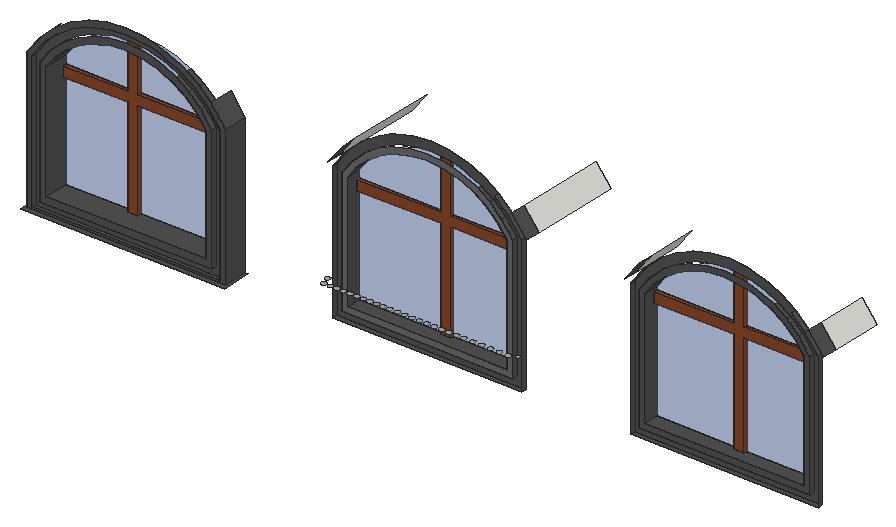
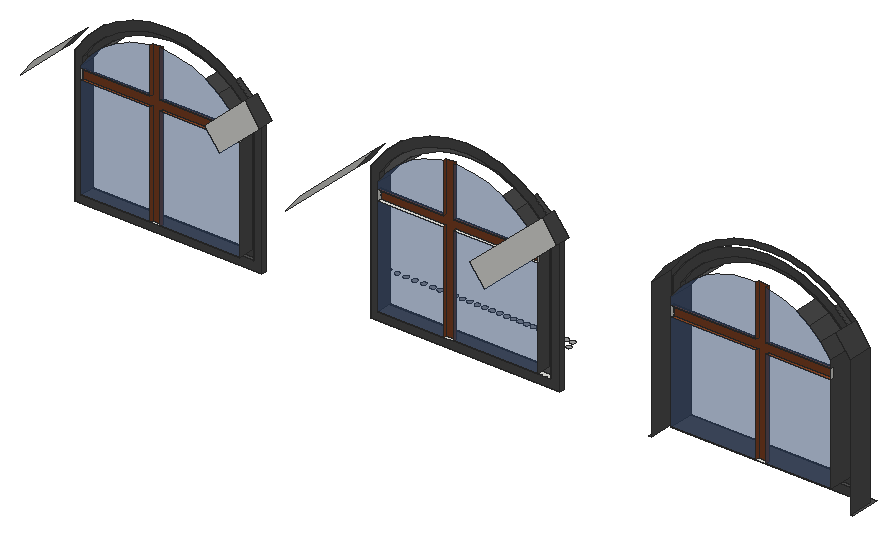
# SketchUp Ruby script. Lengths in inches.
U = 1.inch
M = Sketchup.active_model
def pt(a) = Geom::Point3d.new(a.map { |v| v * U })
def face(e, loops, mat)
  f = e.add_face(loops[0].map { |a| pt(a) })
  loops[1..].each { |l| e.add_face(l.map { |a| pt(a) }).erase! }
  f.material = f.back_material = mat if mat
  f
end
# faces: each face lists its corners as indices into pts; further lists are holes
def faces(e, pts, list, mat = nil) = list.each { |f| face(e, (f[0].is_a?(Array) ? f : [f]).map { |l| l.map { |i| pts[i] } }, mat) }
# xy, xz, yz: faces in a plane at the given z, y or x. An outline is a flat list of corners, or four numbers for a rectangle; further outlines are holes
def ring(l) = l.size == 4 ? [[l[0], l[1]], [l[2], l[1]], [l[2], l[3]], [l[0], l[3]]] : l.each_slice(2).to_a
def flat(e, list, mat, &to3) = list.each { |f| face(e, (f[0].is_a?(Array) ? f : [f]).map { |l| ring(l).map { |u, v| to3.(u, v) } }, mat) }
def xy(e, z, list, mat = nil) = flat(e, list, mat) { |x, y| [x, y, z] }
def xz(e, y, list, mat = nil) = flat(e, list, mat) { |x, z| [x, y, z] }
def yz(e, x, list, mat = nil) = flat(e, list, mat) { |y, z| [x, y, z] }
def lines(e, pts, list) = list.each { |a, b| e.add_line(pt(pts[a]), pt(pts[b])) }
# prism: a flat outline (further loops are holes) pulled along v
def prism(e, loops, v, mat = nil)
  f = face(e, loops, mat); d = Geom::Vector3d.new(v.map { |x| x * U })
  f.pushpull(f.normal.samedirection?(d) ? d.length : -d.length)
end
def box(e, o, s, mat = nil) = prism(e, [[o, [o[0] + s[0], o[1], o[2]], [o[0] + s[0], o[1] + s[1], o[2]], [o[0], o[1] + s[1], o[2]]]], [0, 0, s[2]], mat)
def at(x, y, z, deg = 0) = Geom::Transformation.translation(pt([x, y, z])) * Geom::Transformation.rotation(ORIGIN, Z_AXIS, deg.degrees)
def axes(o, x, y, z) = Geom::Transformation.new([*x, 0, *y, 0, *z, 0, *pt(o).to_a, 1])
def part(name) = M.definitions.add(name)
# library, detail: a bought-in or finely detailed component or shape, given as its bounding box
def library(name, o, s) = part(name).tap { |d| box(d.entities, o, s) }
def detail(e, o, s) = box(e.add_group.entities, o, s)
def put(e, d, t, mat = nil) = e.add_instance(d, t).tap { |i| i.material = mat if mat }
def group(e, t, mat = nil) = e.add_group.tap { |g| g.transformation = t; g.material = mat if mat }.entities
root = M.entities
M.materials.add("[0042_Sienna]").color = [137, 70, 38]
M.materials.add("[0132_LightGray]").color = [169, 169, 169]
M.materials.add("[0134_DimGray]").color = [105, 105, 105]
M.materials.add("[0135_DarkGray]").color = [81, 81, 81]
M.materials.add("[Translucent Glass Blue]").color = [66, 99, 158]
M.materials["[Translucent Glass Blue]"].alpha = 0.5
xy(root,641.05,[[63.64,31.6875,187.39,31.6875,187.39,49.6875,185.57,49.6875,185.57,34.6875,64.89,34.6875,64.89,49.6875,63.64,49.6875]],"[0135_DarkGray]")
xy(root,641.66,[[245.76,40.6875,360.57,43.6875]],"[0135_DarkGray]")
xy(root,641.92,[[68.09,34.6875,182.37,37.6875]],"[0135_DarkGray]")
xy(root,642.07,[[426.42,40.6875,540.41,43.6875]],"[0135_DarkGray]")
xy(root,646.79,[[72.95,34.6875,177.5,37.6875]],"[0135_DarkGray]")
xy(root,647.04,[[251.14,40.6875,355.19,43.6875]])
xy(root,647.27,[[431.625,40.6875,535.21,43.6875]],"[0135_DarkGray]")
xy(root,650.72,[[116.29,47.6875,122.29,49.6875],[305.64,47.6875,311.64,49.6875],[483.7,47.6875,489.7,49.6875]])
xy(root,650.72,[[76.89,34.6875,173.57,34.6875,173.57,49.6875,122.29,49.6875,122.29,47.6875,116.29,47.6875,116.29,49.6875,76.89,49.6875],[254.82,40.6875,351.51,40.6875,351.51,49.6875,311.64,49.6875,311.64,47.6875,305.64,47.6875,305.64,49.6875,254.82,49.6875],[435.07,40.6875,531.76,40.6875,531.76,49.6875,489.7,49.6875,489.7,47.6875,483.7,47.6875,483.7,49.6875,435.07,49.6875]],"[0135_DarkGray]")
xy(root,662.87,[[361.31,35.875,361.57,35.89,361.8125,35.97,362.03,36.11,362.21,36.31,362.32,36.54,362.38,36.8,362.36,37.06,362.28,37.31,362.14,37.52,361.94,37.7,361.71,37.82,361.46,37.87,361.19,37.85,360.95,37.77,360.73,37.63,360.55,37.4375,360.4375,37.2,360.38,36.95,360.4,36.6875,360.48,36.4375,360.62,36.22,360.82,36.05,361.05,35.93]],"[0132_LightGray]")
xy(root,663.85,[[246.33,31.93,246.68,31.97,247.02,32.11,247.3,32.33,247.52,32.62,247.66,32.95,247.7,33.3,247.66,33.66,247.52,33.99,247.3,34.28,247.02,34.49,246.68,34.63,246.33,34.68,245.97,34.63,245.64,34.49,245.36,34.28,245.14,33.99,245,33.66,244.95,33.3,245,32.95,245.14,32.62,245.36,32.33,245.64,32.11,245.97,31.97],[250.33,31.93,250.68,31.97,251.02,32.11,251.3,32.33,251.52,32.62,251.66,32.95,251.7,33.3,251.66,33.66,251.52,33.99,251.3,34.28,251.02,34.49,250.68,34.63,250.33,34.68,249.97,34.63,249.64,34.49,249.36,34.28,249.14,33.99,249,33.66,248.95,33.3,249,32.95,249.14,32.62,249.36,32.33,249.64,32.11,249.97,31.97],[254.33,31.93,254.68,31.97,255.02,32.11,255.3,32.33,255.52,32.62,255.66,32.95,255.7,33.3,255.66,33.66,255.52,33.99,255.3,34.28,255.02,34.49,254.68,34.63,254.33,34.68,253.97,34.63,253.64,34.49,253.36,34.28,253.14,33.99,253,33.66,252.95,33.3,253,32.95,253.14,32.62,253.36,32.33,253.64,32.11,253.97,31.97],[258.33,31.93,258.68,31.97,259.02,32.11,259.3,32.33,259.52,32.62,259.66,32.95,259.7,33.3,259.66,33.66,259.52,33.99,259.3,34.28,259.02,34.49,258.68,34.63,258.33,34.68,257.97,34.63,257.64,34.49,257.36,34.28,257.14,33.99,257,33.66,256.95,33.3,257,32.95,257.14,32.62,257.36,32.33,257.64,32.11,257.97,31.97],[262.33,31.93,262.68,31.97,263.02,32.11,263.3,32.33,263.52,32.62,263.66,32.95,263.7,33.3,263.66,33.66,263.52,33.99,263.3,34.28,263.02,34.49,262.68,34.63,262.33,34.68,261.97,34.63,261.64,34.49,261.36,34.28,261.14,33.99,261,33.66,260.95,33.3,261,32.95,261.14,32.62,261.36,32.33,261.64,32.11,261.97,31.97],
  [266.33,31.93,266.68,31.97,267.02,32.11,267.3,32.33,267.52,32.62,267.66,32.95,267.7,33.3,267.66,33.66,267.52,33.99,267.3,34.28,267.02,34.49,266.68,34.63,266.33,34.68,265.97,34.63,265.64,34.49,265.36,34.28,265.14,33.99,265,33.66,264.95,33.3,265,32.95,265.14,32.62,265.36,32.33,265.64,32.11,265.97,31.97],[270.33,31.93,270.68,31.97,271.02,32.11,271.3,32.33,271.52,32.62,271.66,32.95,271.7,33.3,271.66,33.66,271.52,33.99,271.3,34.28,271.02,34.49,270.68,34.63,270.33,34.68,269.97,34.63,269.64,34.49,269.36,34.28,269.14,33.99,269,33.66,268.95,33.3,269,32.95,269.14,32.62,269.36,32.33,269.64,32.11,269.97,31.97],[274.33,31.93,274.68,31.97,275.02,32.11,275.3,32.33,275.52,32.62,275.66,32.95,275.7,33.3,275.66,33.66,275.52,33.99,275.3,34.28,275.02,34.49,274.68,34.63,274.33,34.68,273.97,34.63,273.64,34.49,273.36,34.28,273.14,33.99,273,33.66,272.95,33.3,273,32.95,273.14,32.62,273.36,32.33,273.64,32.11,273.97,31.97],[278.33,31.93,278.68,31.97,279.02,32.11,279.3,32.33,279.52,32.62,279.66,32.95,279.7,33.3,279.66,33.66,279.52,33.99,279.3,34.28,279.02,34.49,278.68,34.63,278.33,34.68,277.97,34.63,277.64,34.49,277.36,34.28,277.14,33.99,277,33.66,276.95,33.3,277,32.95,277.14,32.62,277.36,32.33,277.64,32.11,277.97,31.97],[282.33,31.93,282.68,31.97,283.02,32.11,283.3,32.33,283.52,32.62,283.66,32.95,283.7,33.3,283.66,33.66,283.52,33.99,283.3,34.28,283.02,34.49,282.68,34.63,282.33,34.68,281.97,34.63,281.64,34.49,281.36,34.28,281.14,33.99,281,33.66,280.95,33.3,281,32.95,281.14,32.62,281.36,32.33,281.64,32.11,281.97,31.97],
  [286.33,31.93,286.68,31.97,287.02,32.11,287.3,32.33,287.52,32.62,287.66,32.95,287.7,33.3,287.66,33.66,287.52,33.99,287.3,34.28,287.02,34.49,286.68,34.63,286.33,34.68,285.97,34.63,285.64,34.49,285.36,34.28,285.14,33.99,285,33.66,284.95,33.3,285,32.95,285.14,32.62,285.36,32.33,285.64,32.11,285.97,31.97],[290.83,31.93,291.18,31.97,291.52,32.11,291.8,32.33,292.02,32.62,292.16,32.95,292.2,33.3,292.16,33.66,292.02,33.99,291.8,34.28,291.52,34.49,291.18,34.63,290.83,34.68,290.47,34.63,290.14,34.49,289.86,34.28,289.64,33.99,289.5,33.66,289.45,33.3,289.5,32.95,289.64,32.62,289.86,32.33,290.14,32.11,290.47,31.97],[295.33,31.93,295.68,31.97,296.02,32.11,296.3,32.33,296.52,32.62,296.66,32.95,296.7,33.3,296.66,33.66,296.52,33.99,296.3,34.28,296.02,34.49,295.68,34.63,295.33,34.68,294.97,34.63,294.64,34.49,294.36,34.28,294.14,33.99,294,33.66,293.95,33.3,294,32.95,294.14,32.62,294.36,32.33,294.64,32.11,294.97,31.97],[299.83,31.93,300.18,31.97,300.52,32.11,300.8,32.33,301.02,32.62,301.16,32.95,301.2,33.3,301.16,33.66,301.02,33.99,300.8,34.28,300.52,34.49,300.18,34.63,299.83,34.68,299.47,34.63,299.14,34.49,298.86,34.28,298.64,33.99,298.5,33.66,298.45,33.3,298.5,32.95,298.64,32.62,298.86,32.33,299.14,32.11,299.47,31.97],[304.33,31.93,304.68,31.97,305.02,32.11,305.3,32.33,305.52,32.62,305.66,32.95,305.7,33.3,305.66,33.66,305.52,33.99,305.3,34.28,305.02,34.49,304.68,34.63,304.33,34.68,303.97,34.63,303.64,34.49,303.36,34.28,303.14,33.99,303,33.66,302.95,33.3,303,32.95,303.14,32.62,303.36,32.33,303.64,32.11,303.97,31.97],
  [308.83,31.93,309.18,31.97,309.52,32.11,309.8,32.33,310.02,32.62,310.16,32.95,310.2,33.3,310.16,33.66,310.02,33.99,309.8,34.28,309.52,34.49,309.18,34.63,308.83,34.68,308.47,34.63,308.14,34.49,307.86,34.28,307.64,33.99,307.5,33.66,307.45,33.3,307.5,32.95,307.64,32.62,307.86,32.33,308.14,32.11,308.47,31.97],[313.33,31.93,313.68,31.97,314.02,32.11,314.3,32.33,314.52,32.62,314.66,32.95,314.7,33.3,314.66,33.66,314.52,33.99,314.3,34.28,314.02,34.49,313.68,34.63,313.33,34.68,312.97,34.63,312.64,34.49,312.36,34.28,312.14,33.99,312,33.66,311.95,33.3,312,32.95,312.14,32.62,312.36,32.33,312.64,32.11,312.97,31.97],[317.83,31.93,318.18,31.97,318.52,32.11,318.8,32.33,319.02,32.62,319.16,32.95,319.2,33.3,319.16,33.66,319.02,33.99,318.8,34.28,318.52,34.49,318.18,34.63,317.83,34.68,317.47,34.63,317.14,34.49,316.86,34.28,316.64,33.99,316.5,33.66,316.45,33.3,316.5,32.95,316.64,32.62,316.86,32.33,317.14,32.11,317.47,31.97],[322.33,31.93,322.68,31.97,323.02,32.11,323.3,32.33,323.52,32.62,323.66,32.95,323.7,33.3,323.66,33.66,323.52,33.99,323.3,34.28,323.02,34.49,322.68,34.63,322.33,34.68,321.97,34.63,321.64,34.49,321.36,34.28,321.14,33.99,321,33.66,320.95,33.3,321,32.95,321.14,32.62,321.36,32.33,321.64,32.11,321.97,31.97],[326.83,31.93,327.18,31.97,327.52,32.11,327.8,32.33,328.02,32.62,328.16,32.95,328.2,33.3,328.16,33.66,328.02,33.99,327.8,34.28,327.52,34.49,327.18,34.63,326.83,34.68,326.47,34.63,326.14,34.49,325.86,34.28,325.64,33.99,325.5,33.66,325.45,33.3,325.5,32.95,325.64,32.62,325.86,32.33,326.14,32.11,326.47,31.97],
  [331.33,31.93,331.68,31.97,332.02,32.11,332.3,32.33,332.52,32.62,332.66,32.95,332.7,33.3,332.66,33.66,332.52,33.99,332.3,34.28,332.02,34.49,331.68,34.63,331.33,34.68,330.97,34.63,330.64,34.49,330.36,34.28,330.14,33.99,330,33.66,329.95,33.3,330,32.95,330.14,32.62,330.36,32.33,330.64,32.11,330.97,31.97],[336.7,31.93,337.06,31.97,337.39,32.11,337.68,32.33,337.89,32.62,338.03,32.95,338.08,33.3,338.03,33.66,337.89,33.99,337.68,34.28,337.39,34.49,337.06,34.63,336.7,34.68,336.35,34.63,336.02,34.49,335.73,34.28,335.51,33.99,335.375,33.66,335.33,33.3,335.375,32.95,335.51,32.62,335.73,32.33,336.02,32.11,336.35,31.97],[342.08,31.93,342.43,31.97,342.77,32.11,343.05,32.33,343.27,32.62,343.41,32.95,343.45,33.3,343.41,33.66,343.27,33.99,343.05,34.28,342.77,34.49,342.43,34.63,342.08,34.68,341.72,34.63,341.39,34.49,341.11,34.28,340.89,33.99,340.75,33.66,340.7,33.3,340.75,32.95,340.89,32.62,341.11,32.33,341.39,32.11,341.72,31.97],[347.45,31.93,347.81,31.97,348.14,32.11,348.43,32.33,348.64,32.62,348.78,32.95,348.83,33.3,348.78,33.66,348.64,33.99,348.43,34.28,348.14,34.49,347.81,34.63,347.45,34.68,347.1,34.63,346.77,34.49,346.48,34.28,346.26,33.99,346.125,33.66,346.08,33.3,346.125,32.95,346.26,32.62,346.48,32.33,346.77,32.11,347.1,31.97],[352.83,31.93,353.18,31.97,353.52,32.11,353.8,32.33,354.02,32.62,354.16,32.95,354.2,33.3,354.16,33.66,354.02,33.99,353.8,34.28,353.52,34.49,353.18,34.63,352.83,34.68,352.47,34.63,352.14,34.49,351.86,34.28,351.64,33.99,351.5,33.66,351.45,33.3,351.5,32.95,351.64,32.62,351.86,32.33,352.14,32.11,352.47,31.97],
  [358.2,31.93,358.56,31.97,358.89,32.11,359.18,32.33,359.39,32.62,359.53,32.95,359.58,33.3,359.53,33.66,359.39,33.99,359.18,34.28,358.89,34.49,358.56,34.63,358.2,34.68,357.85,34.63,357.52,34.49,357.23,34.28,357.01,33.99,356.875,33.66,356.83,33.3,356.875,32.95,357.01,32.62,357.23,32.33,357.52,32.11,357.85,31.97],[244.88,36.8,245.22,36.84,245.53,36.97,245.81,37.18,246.01,37.45,246.15,37.77,246.19,38.11,246.15,38.45,246.01,38.77,245.81,39.04,245.53,39.25,245.22,39.38,244.88,39.42,244.54,39.38,244.22,39.25,243.95,39.04,243.74,38.77,243.61,38.45,243.57,38.11,243.61,37.77,243.74,37.45,243.95,37.18,244.22,36.97,244.54,36.84]],"[0132_LightGray]")
xy(root,710.28,[[76.89,47.6875,116.29,49.6875],[122.29,47.6875,173.57,49.6875]],"[0042_Sienna]")
xy(root,710.91,[[254.82,47.6875,305.64,49.6875],[311.64,47.6875,351.51,49.6875]])
xy(root,713.16,[[435.07,47.6875,483.7,49.6875],[489.7,47.6875,531.76,49.6875]],"[0042_Sienna]")
xy(root,716.28,[[76.89,47.6875,116.29,49.6875],[122.29,47.6875,173.57,49.6875]],"[0042_Sienna]")
xy(root,716.91,[[254.82,47.6875,305.64,49.6875],[311.64,47.6875,351.51,49.6875]],"[0042_Sienna]")
xy(root,719.16,[[435.07,47.6875,483.7,49.6875],[489.7,47.6875,531.76,49.6875]],"[0042_Sienna]")
xz(root,34.6875,[[[64.89,641.05,185.57,641.05,185.57,725.13,176.65,736.74,168.18,744.61,158.52,750.96,151.56,754.04,147.95,755.63,142.09,757.13,136.75,758.49,125.23,759.45,113.71,758.49,108.37,757.13,102.51,755.63,98.9,754.04,91.93,750.96,82.28,744.61,73.8125,736.74,64.89,725.13],[68.09,641.92,68.09,724.05,76.1875,734.58,84.26,742.08,93.47,748.14,100.19,751.11,103.56,752.6,109.16,754.03,114.24,755.32,125.23,756.24,136.22,755.32,141.3,754.03,146.9,752.6,150.27,751.11,156.99,748.14,166.19,742.08,174.27,734.58,182.37,724.05,182.37,641.92]],[[72.95,646.79,177.5,646.79,177.5,722.39,170.66,731.29,163.18,738.24,154.65,743.85,148.3,746.66,145.3,747.98,140.09,749.31,135.41,750.5,125.23,751.35,115.05,750.5,110.36,749.31,105.15,747.98,102.16,746.66,95.81,743.85,87.28,738.24,79.8,731.29,72.95,722.39],[76.89,650.72,76.89,721.05,82.71,728.63,89.72,735.13,97.7,740.39,103.75,743.0625,106.44,744.25,111.33,745.5,115.7,746.61,125.23,747.41,134.75,746.61,139.12,745.5,144.02,744.25,146.71,743.0625,152.76,740.39,160.74,735.13,167.74,728.63,173.57,721.05,173.57,650.72]]],"[0135_DarkGray]")
xz(root,37.6875,[[[68.09,641.92,182.37,641.92,182.37,724.05,174.27,734.58,166.19,742.08,156.99,748.14,150.27,751.11,146.9,752.6,141.3,754.03,136.22,755.32,125.23,756.24,114.24,755.32,109.16,754.03,103.56,752.6,100.19,751.11,93.47,748.14,84.26,742.08,76.1875,734.58,68.09,724.05],[72.95,646.79,72.95,722.39,79.8,731.29,87.28,738.24,95.81,743.85,102.16,746.66,105.15,747.98,110.36,749.31,115.05,750.5,125.23,751.35,135.41,750.5,140.09,749.31,145.3,747.98,148.3,746.66,154.65,743.85,163.18,738.24,170.66,731.29,177.5,722.39,177.5,646.79]]],"[0135_DarkGray]")
xz(root,40.6875,[[[251.14,647.04,355.19,647.04,355.19,722.3,348.41,731.12,340.96,738.04,332.46,743.63,326.14,746.43,323.16,747.74,317.97,749.07,313.3,750.26,303.17,751.1,293.03,750.26,288.36,749.07,283.17,747.74,280.2,746.43,273.87,743.63,265.37,738.04,257.92,731.12,251.14,722.3],[254.82,650.72,254.82,721.05,260.65,728.63,267.65,735.13,275.64,740.39,281.68,743.0625,284.38,744.25,289.27,745.5,293.64,746.61,303.17,747.41,312.69,746.61,317.06,745.5,321.95,744.25,324.65,743.0625,330.7,740.39,338.68,735.13,345.68,728.63,351.51,721.05,351.51,650.72]]],"[0134_DimGray]")
xz(root,40.6875,[[[431.625,647.27,535.21,647.27,535.21,722.22,528.49,730.96,521.06,737.85,512.6,743.43,506.29,746.21,503.33,747.52,498.16,748.84,493.51,750.02,483.42,750.87,473.32,750.02,468.67,748.84,463.5,747.52,460.54,746.21,454.23,743.43,445.77,737.85,438.34,730.96,431.625,722.22],[435.07,650.72,435.07,721.05,440.9,728.63,447.9,735.13,455.89,740.39,461.93,743.0625,464.63,744.25,469.52,745.5,473.89,746.61,483.42,747.41,492.94,746.61,497.31,745.5,502.2,744.25,504.9,743.0625,510.95,740.39,518.93,735.13,525.93,728.63,531.76,721.05,531.76,650.72]]],"[0135_DarkGray]")
xz(root,43.6875,[[[245.76,641.66,360.57,641.66,360.57,724.14,352.41,734.75,344.3,742.29,335.05,748.38,328.3125,751.35,324.92,752.85,319.3,754.28,314.2,755.58,303.17,756.5,292.13,755.58,287.03,754.28,281.41,752.85,278.02,751.35,271.28,748.38,262.04,742.29,253.93,734.75,245.76,724.14],[251.14,647.04,251.14,722.3,257.92,731.12,265.37,738.04,273.87,743.63,280.2,746.43,283.17,747.74,288.36,749.07,293.03,750.26,303.17,751.1,313.3,750.26,317.97,749.07,323.16,747.74,326.14,746.43,332.46,743.63,340.96,738.04,348.41,731.12,355.19,722.3,355.19,647.04]],[[426.42,642.07,540.41,642.07,540.41,724,532.35,734.47,524.29,741.96,515.1,748.01,508.39,750.98,505.04,752.46,499.45,753.88,494.38,755.17,483.42,756.09,472.45,755.17,467.39,753.88,461.79,752.46,458.4375,750.98,451.73,748.01,442.54,741.96,434.48,734.47,426.42,724],[431.625,647.27,431.625,722.22,438.34,730.96,445.77,737.85,454.23,743.43,460.54,746.21,463.5,747.52,468.67,748.84,473.32,750.02,483.42,750.87,493.51,750.02,498.16,748.84,503.33,747.52,506.29,746.21,512.6,743.43,521.06,737.85,528.49,730.96,535.21,722.22,535.21,647.27]]],"[0135_DarkGray]")
xz(root,47.6875,[[116.29,650.72,122.29,650.72,122.29,710.28,173.57,710.28,173.57,716.28,122.29,716.28,122.29,747.16,116.29,746.66,116.29,716.28,76.89,716.28,76.89,710.28,116.29,710.28],[305.64,650.72,311.64,650.72,311.64,710.91,351.51,710.91,351.51,716.91,311.64,716.91,311.64,746.7,305.64,747.2,305.64,716.91,254.82,716.91,254.82,710.91,305.64,710.91],[483.7,650.72,489.7,650.72,489.7,713.16,531.76,713.16,531.76,719.16,489.7,719.16,489.7,746.88,483.7,747.38,483.7,719.16,435.07,719.16,435.07,713.16,483.7,713.16]],"[0042_Sienna]")
xz(root,49.6875,[[76.89,650.72,116.29,710.28],[122.29,650.72,173.57,710.28],[254.82,650.72,305.64,710.91],[311.64,650.72,351.51,710.91],[435.07,650.72,483.7,713.16],
  [489.7,650.72,531.76,713.16],[76.89,716.28,116.29,716.28,116.29,746.66,115.7,746.61,111.33,745.5,106.44,744.25,103.75,743.0625,97.7,740.39,89.72,735.13,82.71,728.63,76.89,721.05],[122.29,716.28,173.57,716.28,173.57,721.05,167.74,728.63,160.74,735.13,152.76,740.39,146.71,743.0625,144.02,744.25,139.12,745.5,134.75,746.61,125.23,747.41,122.29,747.16],[254.82,716.91,305.64,716.91,305.64,747.2,303.17,747.41,293.64,746.61,289.27,745.5,284.38,744.25,281.68,743.0625,275.64,740.39,267.65,735.13,260.65,728.63,254.82,721.05],[311.64,716.91,351.51,716.91,351.51,721.05,345.68,728.63,338.68,735.13,330.7,740.39,324.65,743.0625,321.95,744.25,317.06,745.5,312.69,746.61,311.64,746.7],
  [435.07,719.16,483.7,719.16,483.7,747.38,483.42,747.41,473.89,746.61,469.52,745.5,464.63,744.25,461.93,743.0625,455.89,740.39,447.9,735.13,440.9,728.63,435.07,721.05],[489.7,719.16,531.76,719.16,531.76,721.05,525.93,728.63,518.93,735.13,510.95,740.39,504.9,743.0625,502.2,744.25,497.31,745.5,492.94,746.61,489.7,746.88]],"[Translucent Glass Blue]")
yz(root,64.89,[[34.6875,641.05,49.6875,725.13]],"[0135_DarkGray]")
yz(root,68.09,[[34.6875,641.92,37.6875,724.05]],"[0135_DarkGray]")
yz(root,72.95,[[34.6875,646.79,37.6875,722.39]],"[0135_DarkGray]")
yz(root,76.89,[[47.6875,710.28,49.6875,716.28]])
yz(root,76.89,[[34.6875,650.72,49.6875,650.72,49.6875,710.28,47.6875,710.28,47.6875,716.28,49.6875,716.28,49.6875,721.05,34.6875,721.05]],"[0135_DarkGray]")
yz(root,116.29,[[47.6875,650.72,49.6875,710.28],[47.6875,716.28,49.6875,746.66]],"[0042_Sienna]")
yz(root,122.29,[[47.6875,650.72,49.6875,710.28],[47.6875,716.28,49.6875,747.16]],"[0042_Sienna]")
yz(root,173.57,[[47.6875,710.28,49.6875,716.28]])
yz(root,173.57,[[34.6875,650.72,34.6875,721.05,49.6875,721.05,49.6875,716.28,47.6875,716.28,47.6875,710.28,49.6875,710.28,49.6875,650.72]],"[0135_DarkGray]")
yz(root,177.5,[[34.6875,646.79,37.6875,722.39]],"[0135_DarkGray]")
yz(root,182.37,[[34.6875,641.92,37.6875,724.05]],"[0135_DarkGray]")
yz(root,185.57,[[34.6875,641.05,49.6875,725.13]],"[0135_DarkGray]")
yz(root,245.76,[[40.6875,641.66,43.6875,724.14]],"[0135_DarkGray]")
yz(root,251.14,[[40.6875,647.04,43.6875,722.3]],"[0135_DarkGray]")
yz(root,254.82,[[47.6875,710.91,49.6875,716.91]])
yz(root,254.82,[[40.6875,650.72,49.6875,650.72,49.6875,710.91,47.6875,710.91,47.6875,716.91,49.6875,716.91,49.6875,721.05,40.6875,721.05]],"[0135_DarkGray]")
yz(root,305.64,[[47.6875,650.72,49.6875,710.91],[47.6875,716.91,49.6875,747.2]],"[0042_Sienna]")
yz(root,311.64,[[47.6875,650.72,49.6875,710.91],[47.6875,716.91,49.6875,746.7]],"[0042_Sienna]")
yz(root,351.51,[[47.6875,710.91,49.6875,716.91]])
yz(root,351.51,[[40.6875,650.72,40.6875,721.05,49.6875,721.05,49.6875,716.91,47.6875,716.91,47.6875,710.91,49.6875,710.91,49.6875,650.72]],"[0135_DarkGray]")
yz(root,355.19,[[40.6875,647.04,43.6875,722.3]],"[0135_DarkGray]")
yz(root,360.57,[[40.6875,641.66,43.6875,724.14]],"[0135_DarkGray]")
yz(root,426.42,[[40.6875,642.07,43.6875,724]],"[0135_DarkGray]")
yz(root,431.625,[[40.6875,647.27,43.6875,722.22]],"[0135_DarkGray]")
yz(root,435.07,[[47.6875,713.16,49.6875,719.16]])
yz(root,435.07,[[40.6875,650.72,49.6875,650.72,49.6875,713.16,47.6875,713.16,47.6875,719.16,49.6875,719.16,49.6875,721.05,40.6875,721.05]],"[0135_DarkGray]")
yz(root,483.7,[[47.6875,650.72,49.6875,713.16],[47.6875,719.16,49.6875,747.38]],"[0042_Sienna]")
yz(root,489.7,[[47.6875,650.72,49.6875,713.16],[47.6875,719.16,49.6875,746.88]],"[0042_Sienna]")
yz(root,531.76,[[47.6875,713.16,49.6875,719.16]])
yz(root,531.76,[[40.6875,650.72,40.6875,721.05,49.6875,721.05,49.6875,719.16,47.6875,719.16,47.6875,713.16,49.6875,713.16,49.6875,650.72]],"[0135_DarkGray]")
yz(root,535.21,[[40.6875,647.27,43.6875,722.22]],"[0135_DarkGray]")
yz(root,540.41,[[40.6875,642.07,43.6875,724]],"[0135_DarkGray]")
p = [[76.89,49.6875,721.05],[82.71,49.6875,728.63],[82.71,34.6875,728.63],[76.89,34.6875,721.05],[167.74,49.6875,728.63],[173.57,49.6875,721.05],
  [173.57,34.6875,721.05],[167.74,34.6875,728.63],[254.82,49.6875,721.05],[260.65,49.6875,728.63],[260.65,40.6875,728.63],[254.82,40.6875,721.05],
  [345.68,49.6875,728.63],[351.51,49.6875,721.05],[351.51,40.6875,721.05],[345.68,40.6875,728.63],[435.07,49.6875,721.05],[440.9,49.6875,728.63],
  [440.9,40.6875,728.63],[435.07,40.6875,721.05],[525.93,49.6875,728.63],[531.76,49.6875,721.05],[531.76,40.6875,721.05],[525.93,40.6875,728.63],
  [438.34,43.6875,730.96],[431.625,43.6875,722.22],[431.625,40.6875,722.22],[438.34,40.6875,730.96],[535.21,43.6875,722.22],[528.49,43.6875,730.96],
  [528.49,40.6875,730.96],[535.21,40.6875,722.22],[257.92,43.6875,731.12],[251.14,43.6875,722.3],[251.14,40.6875,722.3],[257.92,40.6875,731.12],
  [355.19,43.6875,722.3],[348.41,43.6875,731.12],[348.41,40.6875,731.12],[355.19,40.6875,722.3],[79.8,37.6875,731.29],[72.95,37.6875,722.39],
  [72.95,34.6875,722.39],[79.8,34.6875,731.29],[177.5,37.6875,722.39],[170.66,37.6875,731.29],[170.66,34.6875,731.29],[177.5,34.6875,722.39],
  [68.09,37.6875,724.05],[76.1875,37.6875,734.58],[76.1875,34.6875,734.58],[68.09,34.6875,724.05],[174.27,37.6875,734.58],[182.37,37.6875,724.05],
  [182.37,34.6875,724.05],[174.27,34.6875,734.58],[426.42,43.6875,724],[434.48,43.6875,734.47],[434.48,40.6875,734.47],[426.42,40.6875,724],
  [532.35,43.6875,734.47],[540.41,43.6875,724],[540.41,40.6875,724],[532.35,40.6875,734.47],[245.76,43.6875,724.14],[253.93,43.6875,734.75],
  [253.93,40.6875,734.75],[245.76,40.6875,724.14],[352.41,43.6875,734.75],[360.57,43.6875,724.14],[360.57,40.6875,724.14],[352.41,40.6875,734.75],
  [73.8125,49.6875,736.74],[64.89,49.6875,725.13],[64.89,34.6875,725.13],[73.8125,34.6875,736.74],[185.57,49.6875,725.13],[176.65,49.6875,736.74],
  [176.65,34.6875,736.74],[185.57,34.6875,725.13],[251.75,49.6875,736.74],[242.82,49.6875,725.13],[242.82,40.6875,725.13],[251.75,40.6875,736.74],
  [363.51,49.6875,725.13],[354.58,49.6875,736.74],[354.58,40.6875,736.74],[363.51,40.6875,725.13],[423.07,49.6875,725.13],[432,49.6875,736.74],
  [432,40.6875,736.74],[423.07,40.6875,725.13],[534.83,49.6875,736.74],[543.76,49.6875,725.13],[543.76,40.6875,725.13],[534.83,40.6875,736.74],
  [242.82,104.375,725.13],[251.75,104.375,736.74],[354.58,104.375,736.74],[363.51,104.375,725.13],[423.07,80.4375,725.13],[432,80.4375,736.74],
  [534.83,80.4375,736.74],[543.76,80.4375,725.13],[89.72,49.6875,735.13],[89.72,34.6875,735.13],[160.74,49.6875,735.13],[160.74,34.6875,735.13],
  [267.65,49.6875,735.13],[267.65,40.6875,735.13],[338.68,49.6875,735.13],[338.68,40.6875,735.13],[447.9,49.6875,735.13],[447.9,40.6875,735.13],
  [518.93,49.6875,735.13],[518.93,40.6875,735.13],[445.77,43.6875,737.85],[445.77,40.6875,737.85],[521.06,43.6875,737.85],[521.06,40.6875,737.85],
  [265.37,43.6875,738.04],[265.37,40.6875,738.04],[340.96,43.6875,738.04],[340.96,40.6875,738.04],[87.28,37.6875,738.24],[87.28,34.6875,738.24],
  [163.18,37.6875,738.24],[163.18,34.6875,738.24],[442.54,43.6875,741.96],[442.54,40.6875,741.96],[524.29,43.6875,741.96],[524.29,40.6875,741.96],
  [84.26,37.6875,742.08],[84.26,34.6875,742.08],[166.19,37.6875,742.08],[166.19,34.6875,742.08],[262.04,43.6875,742.29],[262.04,40.6875,742.29],
  [344.3,43.6875,742.29],[344.3,40.6875,742.29],[97.7,49.6875,740.39],[97.7,34.6875,740.39],[152.76,49.6875,740.39],[152.76,34.6875,740.39],
  [275.64,49.6875,740.39],[275.64,40.6875,740.39],[330.7,49.6875,740.39],[330.7,40.6875,740.39],[455.89,49.6875,740.39],[455.89,40.6875,740.39],
  [510.95,49.6875,740.39],[510.95,40.6875,740.39]]
faces(root,p,[[0,1,2,3],[4,5,6,7],[8,9,10,11],[12,13,14,15],[16,17,18,19],[20,21,22,23],[24,25,26,27],[28,29,30,31],
  [32,33,34,35],[36,37,38,39],[40,41,42,43],[44,45,46,47],[48,49,50,51],[52,53,54,55],[56,57,58,59],[60,61,62,63],
  [64,65,66,67],[68,69,70,71],[72,73,74,75],[76,77,78,79],[80,81,82,83],[84,85,86,87],[88,89,90,91],[92,93,94,95],
  [1,104,105,2],[106,4,7,107],[9,108,109,10],[110,12,15,111],[17,112,113,18],[114,20,23,115],[116,24,27,117],[29,118,119,30],
  [120,32,35,121],[37,122,123,38],[124,40,43,125],[45,126,127,46],[57,128,129,58],[130,60,63,131],[49,132,133,50],[134,52,55,135],
  [65,136,137,66],[138,68,71,139],[104,140,141,105],[142,106,107,143],[108,144,145,109],[146,110,111,147],[112,148,149,113],[150,114,115,151]],"[0135_DarkGray]")
faces(root,p,[[80,81,96,97],[84,85,98,99],[89,88,100,101],[93,92,102,103]])
